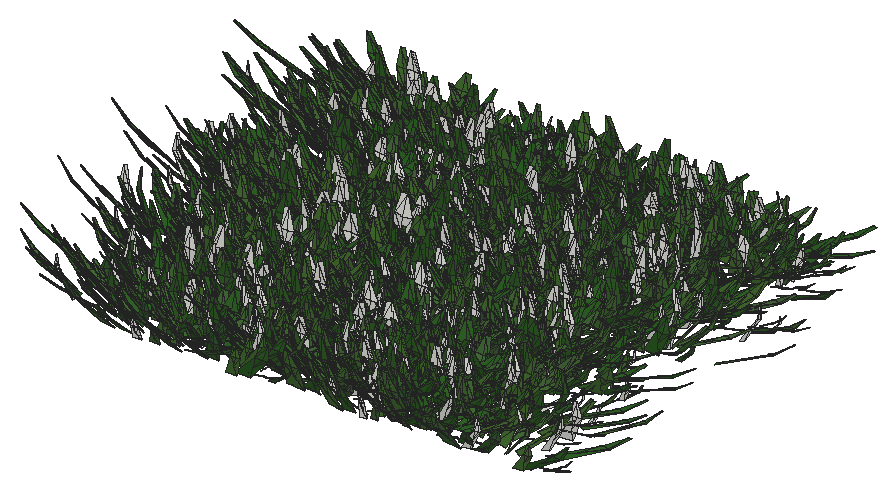
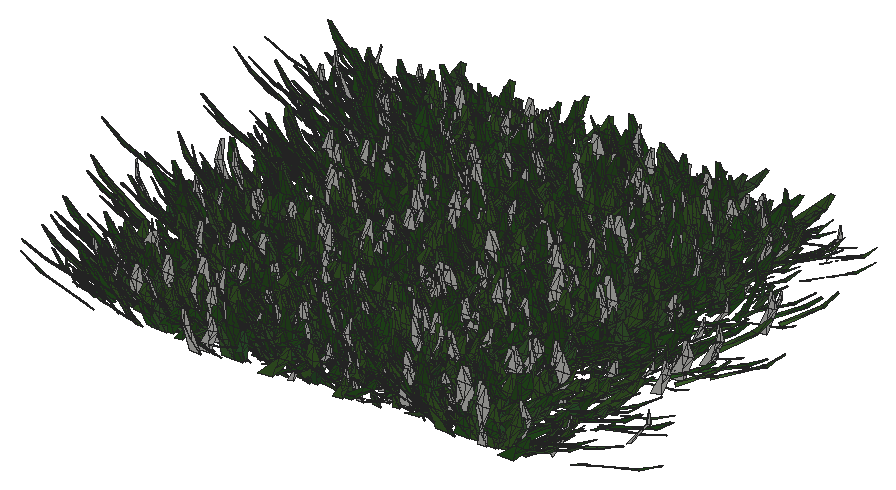
# SketchUp Ruby script. Lengths in inches.
U = 1.inch
M = Sketchup.active_model
def pt(a) = Geom::Point3d.new(a.map { |v| v * U })
def face(e, loops, mat)
  f = e.add_face(loops[0].map { |a| pt(a) })
  loops[1..].each { |l| e.add_face(l.map { |a| pt(a) }).erase! }
  f.material = f.back_material = mat if mat
  f
end
# faces: each face lists its corners as indices into pts; further lists are holes
def faces(e, pts, list, mat = nil) = list.each { |f| face(e, (f[0].is_a?(Array) ? f : [f]).map { |l| l.map { |i| pts[i] } }, mat) }
# xy, xz, yz: faces in a plane at the given z, y or x. An outline is a flat list of corners, or four numbers for a rectangle; further outlines are holes
def ring(l) = l.size == 4 ? [[l[0], l[1]], [l[2], l[1]], [l[2], l[3]], [l[0], l[3]]] : l.each_slice(2).to_a
def flat(e, list, mat, &to3) = list.each { |f| face(e, (f[0].is_a?(Array) ? f : [f]).map { |l| ring(l).map { |u, v| to3.(u, v) } }, mat) }
def xy(e, z, list, mat = nil) = flat(e, list, mat) { |x, y| [x, y, z] }
def xz(e, y, list, mat = nil) = flat(e, list, mat) { |x, z| [x, y, z] }
def yz(e, x, list, mat = nil) = flat(e, list, mat) { |y, z| [x, y, z] }
def lines(e, pts, list) = list.each { |a, b| e.add_line(pt(pts[a]), pt(pts[b])) }
# prism: a flat outline (further loops are holes) pulled along v
def prism(e, loops, v, mat = nil)
  f = face(e, loops, mat); d = Geom::Vector3d.new(v.map { |x| x * U })
  f.pushpull(f.normal.samedirection?(d) ? d.length : -d.length)
end
def box(e, o, s, mat = nil) = prism(e, [[o, [o[0] + s[0], o[1], o[2]], [o[0] + s[0], o[1] + s[1], o[2]], [o[0], o[1] + s[1], o[2]]]], [0, 0, s[2]], mat)
def at(x, y, z, deg = 0) = Geom::Transformation.translation(pt([x, y, z])) * Geom::Transformation.rotation(ORIGIN, Z_AXIS, deg.degrees)
def axes(o, x, y, z) = Geom::Transformation.new([*x, 0, *y, 0, *z, 0, *pt(o).to_a, 1])
def part(name) = M.definitions.add(name)
# library, detail: a bought-in or finely detailed component or shape, given as its bounding box
def library(name, o, s) = part(name).tap { |d| box(d.entities, o, s) }
def detail(e, o, s) = box(e.add_group.entities, o, s)
def put(e, d, t, mat = nil) = e.add_instance(d, t).tap { |i| i.material = mat if mat }
def group(e, t, mat = nil) = e.add_group.tap { |g| g.transformation = t; g.material = mat if mat }.entities
root = M.entities
M.materials.add("Material10").color = [48, 100, 38]
M.materials.add("Material3").color = [68, 110, 58]
M.materials.add("Material4").color = [48, 90, 38]
M.materials.add("Material5").color = [68, 110, 48]
M.materials.add("Material6").color = [48, 90, 48]
M.materials.add("Material7").color = [58, 110, 58]
M.materials.add("Material8").color = [58, 90, 38]
M.materials.add("Material9").color = [68, 100, 58]
c1 = part("grass00")
p = [[-0.6875,0.15,0],[-0.56,0.08,5.52],[-0.04,0.03,2.76],[0.48,-0.02,0],[0.35,-0.02,5.52],[-0.1,-0.14,5.52],
  [-0.12,0.65,8.37],[-0.42,0.65,8.37]]
faces(c1.entities,p,[[0,1,2,3],[3,2,4],[1,5,2],[5,4,2],[1,6,5],[4,5,6],[7,6,1]])
c2 = part("Group16\#1")
put(c2.entities,c1,axes([1.44,-0.61,-0.01],[0.05352,0.12609,0],[-0.10704,0.04543,0.07239],[0.06664,-0.02828,0.11628]),"Material6")
put(c2.entities,c1,axes([0.76,-0.15,-0.01],[0.04676,0.24062,0],[-0.23162,0.04501,0.06642],[0.0652,-0.01267,0.23595]),"Material3")
put(c2.entities,c1,axes([0.79,0.01,-0.01],[-0.00606,0.34651,0],[-0.34381,-0.00602,0.0432],[0.04319,0.00076,0.34386]))
put(c2.entities,c1,axes([1,0.23,-0.01],[-0.07192,0.31144,0],[-0.28722,-0.06632,0.1236],[0.12043,0.02781,0.29478]),"Material5")
put(c2.entities,c1,axes([1.66,0.77,-0.01],[-0.13828,0.29651,0],[-0.21551,-0.1005,0.22471],[0.20365,0.09498,0.23779]),"Material10")
put(c2.entities,c1,axes([0.6875,0.52,-0.01],[-0.18126,0.24051,0],[-0.22746,-0.17142,0.09788],[0.07817,0.05891,0.28481]),"Material5")
put(c2.entities,c1,axes([0.68,0.78,-0.01],[-0.215,0.18688,0],[-0.12385,-0.14248,0.21334],[0.13995,0.16101,0.18878]),"Material3")
put(c2.entities,c1,axes([0.56,1,-0.01],[-0.13756,0.07624,0],[-0.06159,-0.11112,0.0927],[0.04494,0.08108,0.12705]),"Material5")
put(c2.entities,c1,axes([0.2,0.64,-0.01],[-0.23729,0.07254,0],[-0.05711,-0.18681,0.153],[0.04473,0.14632,0.19535]),"Material10")
put(c2.entities,c1,axes([0.0625,0.72,-0.01],[-0.28874,0.02525,0],[-0.02179,-0.24916,0.14647],[0.01276,0.14591,0.25012]),"Material3")
put(c2.entities,c1,axes([-0.08,0.62,-0.01],[-0.34089,-0.04187,0],[0.03255,-0.26504,0.216],[-0.02633,0.21439,0.26703]),"Material10")
put(c2.entities,c1,axes([-0.34,0.98,-0.01],[-0.14314,-0.0493,0],[0.04397,-0.12769,0.06843],[-0.02228,0.0647,0.13505]),"Material10")
put(c2.entities,c1,axes([-0.87,1.45,-0.01],[-0.23488,-0.14114,0],[0.13761,-0.22901,0.06087],[-0.03135,0.05217,0.26717]))
put(c2.entities,c1,axes([-0.72,0.77,-0.01],[-0.14208,-0.13251,0],[0.07209,-0.0773,0.16301],[-0.11118,0.11922,0.1057]),"Material10")
put(c2.entities,c1,axes([-0.62,0.43,-0.01],[-0.14845,-0.21203,0],[0.18654,-0.13061,0.12304],[-0.10079,0.07057,0.22772]),"Material3")
put(c2.entities,c1,axes([-0.68,0.29,-0.01],[-0.13639,-0.32136,0],[0.31723,-0.13464,0.05579],[-0.05136,0.0218,0.34462]),"Material4")
put(c2.entities,c1,axes([-0.64,0.125,-0.01],[-0.0458,-0.23569,0],[0.22124,-0.043,0.08276],[-0.08124,0.01579,0.22538]),"Material7")
put(c2.entities,c1,axes([-1.6,-0.03,-0.01],[0.00576,-0.32897,0],[0.27526,0.00482,0.18018],[-0.18015,-0.00315,0.2753]),"Material5")
put(c2.entities,c1,axes([-1.36,-0.31,-0.01],[0.05718,-0.24765,0],[0.18172,0.04196,0.17267],[-0.16825,-0.03885,0.1865]),"Material10")
put(c2.entities,c1,axes([-1.54,-0.72,-0.01],[0.06537,-0.14017,0],[0.13555,0.06321,0.03939],[-0.0357,-0.01665,0.14956]))
put(c2.entities,c1,axes([-1.19,-0.9,-0.01],[0.09597,-0.12735,0],[0.11214,0.08451,0.07557],[-0.06035,-0.04548,0.14042]),"Material9")
put(c2.entities,c1,axes([-0.47,-0.54,-0.01],[0.11588,-0.10072,0],[0.0618,0.0711,0.12124],[-0.07953,-0.0915,0.0942]))
put(c2.entities,c1,axes([-0.47,-0.84,-0.01],[0.11927,-0.0661,0],[0.06603,0.11913,0.00646],[-0.00313,-0.00565,0.13621]),"Material5")
put(c2.entities,c1,axes([-0.38,-1.24,-0.01],[0.28037,-0.08571,0],[0.0618,0.20215,0.20315],[-0.05939,-0.19428,0.21139]),"Material9")
put(c2.entities,c1,axes([-0.06,-0.66,-0.01],[0.22719,-0.01987,0],[0.01247,0.14255,0.17758],[-0.01547,-0.17691,0.1431]),"Material8")
put(c2.entities,c1,axes([0.11,-0.89,-0.01],[0.14882,0.01828,0],[-0.01058,0.08611,0.12229],[0.01491,-0.12138,0.08676]),"Material6")
put(c2.entities,c1,axes([0.25,-0.72,-0.01],[0.20481,0.07053,0],[-0.06206,0.18022,0.10291],[0.03351,-0.0973,0.1906]),"Material6")
put(c2.entities,c1,axes([0.85,-1.42,-0.01],[0.16481,0.09904,0],[-0.09472,0.15762,0.05616],[0.02893,-0.04814,0.18389]),"Material5")
put(c2.entities,c1,axes([1.01,-1.09,-0.01],[0.21858,0.20385,0],[-0.17495,0.1876,0.15339],[0.10462,-0.11218,0.25652]),"Material10")
put(c2.entities,c1,axes([1.01,-0.71,-0.01],[0.08733,0.12473,0],[-0.06445,0.04512,0.13037],[0.1068,-0.07477,0.07867]),"Material6")
c3 = part("Group15\#1")
put(c3.entities,c2,at(0,0,0))
c4 = part("3darcstudiotree_grass00\#1")
put(c4.entities,c3,at(0,0,0))
put(root,c4,axes([1060.05,905.06,0],[3.81718,0.38538,0],[-1.70529,1.05566,-0.03343],[-0.08298,0.05137,1.88641]))
put(root,c4,axes([1060.56,931.82,0],[-0.16779,1.03236,0],[-3.91072,-0.03973,-0.03031],[-0.21719,-0.00221,1.75443]))
put(root,c4,axes([1060.23,917.13,0],[3.62954,0.33152,0],[-1.65878,1.13506,-0.04863],[-0.08609,0.05891,1.5585]))
put(root,c4,axes([1061.57,930.84,0],[-4.32193,0.57757,0],[-2.28366,-1.06804,-0.02635],[-0.05701,-0.02666,1.3895]))
put(root,c4,axes([1060.06,925.65,0],[2.41826,1.00361,0],[-4.45314,0.67064,-0.01693],[-0.07141,0.01075,1.59984]))
put(root,c4,axes([1060.86,914.74,0],[4.97151,0.37477,0],[-1.19031,0.98689,-0.04516],[-0.09125,0.07566,1.80387]))
put(root,c4,axes([1061.64,923.72,0],[-2.49241,1.02032,0],[-4.21954,-0.64421,-0.0342],[-0.15461,-0.0236,1.63693]))
put(root,c4,axes([1061.28,912.34,0],[3.70549,0.72715,0],[-2.49617,0.79502,-0.02005],[-0.09119,0.02904,1.86077]))
put(root,c4,axes([1063.53,931.57,0],[0.01218,-1.00906,0],[4.98185,0.00376,-0.03692],[0.18714,0.00014,1.57831]))
put(root,c4,axes([1063.89,916.37,0],[-1.42025,-0.83489,0],[4.16242,-0.44255,-0.01791],[0.11075,-0.01178,1.89984]))
put(root,c4,axes([1064.01,901.35,0],[0.28027,-0.96199,0],[3.64955,0.06646,-0.00937],[0.0792,0.00144,1.93766]))
put(root,c4,axes([1063.89,898.16,0],[-3.43805,0.34453,0],[-1.648,-1.02783,-0.04281],[-0.10438,-0.0651,1.81418]))
put(root,c4,axes([1063.77,927.84,0],[3.40925,-0.75567,0],[3.0298,0.85432,-0.03392],[0.10448,0.02946,1.32537]))
put(root,c4,axes([1064.98,905.9,0],[-4.27926,0.10077,0],[-0.4125,-1.0948,-0.0202],[-0.01348,-0.03577,1.95637]))
put(root,c4,axes([1063.73,894.94,0],[3.9837,-0.03206,0],[0.11597,0.90077,-0.04101],[0.00803,0.06239,1.37186]))
put(root,c4,axes([1064.41,930.31,0],[-2.74206,0.64257,0],[-3.29567,-0.87899,-0.02311],[-0.07278,-0.01941,1.38694]))
put(root,c4,axes([1065.68,925.63,0],[-4.52462,0.16915,0],[-0.75823,-1.26762,-0.06496],[-0.05656,-0.09455,1.88637]))
put(root,c4,axes([1064.79,913.76,0],[-1.87065,0.77621,0],[-4.34622,-0.65464,-0.04504],[-0.23728,-0.03574,1.9506]))
put(root,c4,axes([1065,920.09,0],[4.16044,-0.73269,0],[2.40364,0.85303,-0.03692],[0.14968,0.05312,1.83631]))
put(root,c4,axes([1064.86,896.66,0],[3.59915,0.14594,0],[-0.59052,0.91023,-0.01255],[-0.01426,0.02198,1.63564]))
put(root,c4,axes([1065.52,924.38,0],[-2.60039,0.90097,0],[-2.99223,-0.53976,-0.00844],[-0.04191,-0.00756,1.41311]))
put(root,c4,axes([1064.78,918.18,0],[2.59672,0.84047,0],[-3.92214,0.75737,-0.04605],[-0.16947,0.03272,1.44046]))
put(root,c4,axes([1066.125,907.85,0],[1.82286,-0.79645,0],[3.62821,0.519,-0.04415],[0.29175,0.04173,1.98924]))
put(root,c4,axes([1067.33,928.83,0],[-0.69021,-1.10068,0],[5.10027,-0.19989,-0.06318],[0.26987,-0.01058,1.39517]))
put(root,c4,axes([1065.64,908.85,0],[2.76483,1.10064,0],[-3.85856,0.6058,-0.052],[-0.27462,0.04312,1.7759]))
put(root,c4,axes([1066.5,923.28,0],[3.65122,-0.89135,0],[3.24538,0.83087,-0.04175],[0.1632,0.04178,1.62422]))
put(root,c4,axes([1065.84,920.87,0],[4.36658,0.08239,0],[-0.38033,1.25977,-0.00004],[-0.00002,0.00006,1.93334]))
put(root,c4,axes([1067.64,903.13,0],[-2.28283,-1.06843,0],[4.21309,-0.56261,-0.05822],[0.33198,-0.04433,1.92982]))
put(root,c4,axes([1066.68,914.86,0],[0.26997,1.23611,0],[-4.58463,0.06258,-0.05861],[-0.40129,0.00548,1.96776]))
put(root,c4,axes([1066.15,911.15,0],[4.48895,0.48675,0],[-1.69756,0.97846,-0.01845],[-0.03711,0.02139,1.34771]))
put(root,c4,axes([1066.18,894.22,0],[2.13817,1.11793,0],[-4.20741,0.50295,-0.01048],[-0.04572,0.00547,1.40926]))
put(root,c4,axes([1066.53,904.47,0],[4.31033,0.25907,0],[-1.20979,1.25799,-0.03506],[-0.03358,0.03491,1.32515]))
put(root,c4,axes([1067.25,900.07,0],[4.12313,-0.24157,0],[1.18082,1.25966,-0.02268],[0.02474,0.0264,1.5468]))
put(root,c4,axes([1067.24,911.875,0],[-0.03316,1.25701,0],[-4.94993,-0.00816,-0.01347],[-0.06338,-0.0001,1.45625]))
put(root,c4,axes([1069.67,899.01,0],[3.15531,-0.58243,0],[2.70786,0.91686,-0.02283],[0.06907,0.02339,1.4512]))
put(root,c4,axes([1070.67,902.47,0],[-1.85827,-1.20054,0],[4.6379,-0.44867,-0.05475],[0.3098,-0.02997,1.88574]))
put(root,c4,axes([1069.67,897,0],[3.52758,-0.61527,0],[2.26758,0.81256,-0.00731],[0.03042,0.0109,1.80073]))
put(root,c4,axes([1070.9,931.73,0],[-2.08937,-0.99009,0],[3.80908,-0.50239,-0.03938],[0.17969,-0.0237,1.38871]))
put(root,c4,axes([1069.88,922.42,0],[3.90144,-0.65649,0],[2.04826,0.76078,-0.0013],[0.00472,0.00175,1.49257]))
put(root,c4,axes([1069.77,904.9,0],[-1.15605,0.94536,0],[-4.28561,-0.32755,-0.0271],[-0.16007,-0.01223,1.72974]))
put(root,c4,axes([1071.1875,899.8125,0],[-4.45544,0.35262,0],[-1.28974,-1.0185,-0.03323],[-0.0666,-0.05259,1.77353]))
put(root,c4,axes([1070.16,895.2,0],[4.66445,0.12304,0],[-0.40469,0.95886,-0.03171],[-0.02368,0.05611,1.71518]))
put(root,c4,axes([1071.92,906.49,0],[0.22891,-1.1855,0],[4.26581,0.05148,-0.00402],[0.01994,0.00024,1.3243]))
put(root,c4,axes([1072.04,910.74,0],[-3.83276,-0.4307,0],[1.47756,-0.82179,-0.02079],[0.061,-0.03393,1.61237]))
put(root,c4,axes([1071.23,912.24,0],[-2.46367,0.88426,0],[-3.17691,-0.55321,-0.01437],[-0.09353,-0.01629,1.91898]))
put(root,c4,axes([1072.21,927.79,0],[-2.3426,-0.88357,0],[3.5724,-0.59197,-0.05028],[0.30493,-0.05053,1.94898]))
put(root,c4,axes([1070.97,930.54,0],[4.40447,-0.22368,0],[0.75254,0.92613,-0.00331],[0.00443,0.00545,1.58887]))
put(root,c4,axes([1070.42,921.03,0],[4.73855,0.38676,0],[-1.49783,1.14695,-0.00124],[-0.0021,0.00161,1.65228]))
put(root,c4,axes([1071.73,926.16,0],[-1.79093,0.80578,0],[-3.73339,-0.51862,-0.05151],[-0.32129,-0.04463,1.90487]))
put(root,c4,axes([1070.86,924.13,0],[1.1144,0.95521,0],[-4.67069,0.34057,-0.00405],[-0.01733,0.00126,1.35389]))
put(root,c4,axes([1073.37,918.5,0],[-3.69018,-0.70839,0],[2.67455,-0.87078,-0.00705],[0.02875,-0.00936,1.8369]))
put(root,c4,axes([1072.42,919.6,0],[2.21238,-0.82212,0],[4.12079,0.69308,-0.06298],[0.2244,0.03774,1.33293]))
put(root,c4,axes([1071.57,894.17,0],[4.71925,-0.11324,0],[0.46781,1.21853,-0.01064],[0.0059,0.01536,1.77558]))
put(root,c4,axes([1073.51,929.0625,0],[-3.23059,-0.98889,0],[3.90689,-0.79771,-0.03335],[0.15229,-0.03109,1.85855]))
put(root,c4,axes([1072.875,915.7,0],[0.38736,-1.28995,0],[5.0857,0.09545,-0.06273],[0.38626,0.00725,1.9684]))
put(root,c4,axes([1072.43,901.1,0],[-1.91482,0.78597,0],[-3.52393,-0.53658,-0.03041],[-0.133,-0.02025,1.3205]))
put(root,c4,axes([1073.875,914.15,0],[-1.97779,-0.85605,0],[3.47193,-0.50134,-0.00817],[0.04391,-0.00634,1.55447]))
put(root,c4,axes([1073.05,916.17,0],[4.07935,-0.43346,0],[1.89845,1.11667,-0.00549],[0.0102,0.006,1.44062]))
put(root,c4,axes([1073.04,907.98,0],[4.37754,-0.30034,0],[1.33809,1.21894,-0.05143],[0.06212,0.05659,1.44218]))
put(root,c4,axes([1073,909.25,0],[-0.77459,1.02893,0],[-4.84534,-0.22797,-0.01956],[-0.11313,-0.00532,1.8138]))
put(root,c4,axes([1075.72,906.38,0],[-4.74279,0.28772,0],[-1.21823,-1.25511,-0.06662],[-0.06794,-0.07,1.39642]))
put(root,c4,axes([1076.68,899.54,0],[-3.58073,-0.35661,0],[1.83074,-1.1489,-0.00121],[0.00279,-0.00175,1.92636]))
put(root,c4,axes([1075.85,930.3125,0],[1.54312,-0.81512,0],[3.29472,0.38983,-0.04441],[0.34585,0.04092,1.96303]))
put(root,c4,axes([1076.66,927.34,0],[-0.36487,-0.9693,0],[3.80087,-0.08942,-0.04952],[0.26852,-0.00632,1.29958]))
put(root,c4,axes([1076.78,924.32,0],[-3.87388,0.80913,0],[-2.80413,-0.83909,-0.03098],[-0.11588,-0.03468,1.59479]))
put(root,c4,axes([1077.45,932.95,0],[-4.21097,-0.15572,0],[0.54772,-0.92572,-0.00812],[0.00706,-0.01193,1.3892]))
put(root,c4,axes([1076.93,920.93,0],[-3.28993,0.53414,0],[-2.35898,-0.90811,-0.04277],[-0.16039,-0.06174,1.86401]))
put(root,c4,axes([1076.34,901.25,0],[-0.64164,1.09647,0],[-3.76994,-0.13788,-0.02144],[-0.17386,-0.00636,1.9513]))
put(root,c4,axes([1076.9,915.71,0],[-3.33719,0.61695,0],[-2.63683,-0.89144,-0.01371],[-0.03862,-0.01306,1.31321]))
put(root,c4,axes([1076.34,929.21,0],[3.65959,-0.0096,0],[0.04442,1.05836,-0.01029],[0.00057,0.0135,1.389]))
put(root,c4,axes([1077.57,904.44,0],[1.63627,-0.81784,0],[3.89049,0.48648,-0.01805],[0.09406,0.01176,1.58457]))
put(root,c4,axes([1076.61,919.86,0],[4.2926,-0.51485,0],[1.76165,0.91799,-0.04597],[0.12323,0.06421,1.57738]))
put(root,c4,axes([1076.81,917.96,0],[-2.40518,0.923,0],[-4.34744,-0.70804,-0.00953],[-0.03635,-0.00592,1.47621]))
put(root,c4,axes([1078.18,931.99,0],[1.06062,-0.94983,0],[4.26034,0.29733,-0.00232],[0.01421,0.00099,1.76107]))
put(root,c4,axes([1077.08,922.95,0],[3.58152,-0.18688,0],[0.799,0.95704,-0.04941],[0.06002,0.07189,1.4533]))
put(root,c4,axes([1078.43,911.17,0],[2.30537,-0.84658,0],[3.6231,0.61664,-0.01892],[0.09951,0.01694,1.74337]))
put(root,c4,axes([1078.3,896.47,0],[-2.37312,0.89049,0],[-3.32471,-0.55376,-0.03773],[-0.17795,-0.02964,1.41517]))
put(root,c4,axes([1077.45,925.65,0],[4.42223,0.30333,0],[-1.18434,1.07915,-0.02738],[-0.04878,0.04444,1.88342]))
put(root,c4,axes([1078.06,916.16,0],[4.7526,-0.49648,0],[1.99217,1.19189,-0.05614],[0.10535,0.06303,1.57175]))
put(root,c4,axes([1079.17,908.06,0],[2.12632,-1.16665,0],[4.03974,0.46017,-0.02827],[0.17992,0.0205,1.94019]))
put(root,c4,axes([1078.41,912.15,0],[0.82616,1.18847,0],[-3.57688,0.1554,-0.03272],[-0.26216,0.01139,1.8454]))
put(root,c4,axes([1078.12,913.71,0],[3.22998,0.67416,0],[-3.0562,0.91516,-0.05497],[-0.20916,0.06263,1.76958]))
put(root,c4,axes([1078.09,908.5625,0],[2.39946,0.73907,0],[-3.00526,0.6098,-0.00448],[-0.02213,0.00449,1.5389]))
put(root,c4,axes([1079.36,903.23,0],[2.55238,-0.83938,0],[4.10588,0.78031,-0.05929],[0.21983,0.04178,1.50135]))
put(root,c4,axes([1079.08,895.41,0],[-0.55541,1.00886,0],[-4.55532,-0.15674,-0.0385],[-0.20653,-0.00711,1.55608]))
put(root,c4,axes([1079.5,898.66,0],[4.68045,-0.41888,0],[1.5867,1.1081,-0.05713],[0.0969,0.06767,1.48067]))
put(root,c4,axes([1081.74,925.4,0],[-3.20384,-1.02326,0],[3.97726,-0.7783,-0.01534],[0.06587,-0.01289,1.72134]))
put(root,c4,axes([1081.51,915.32,0],[-4.59803,0.08563,0],[-0.2847,-0.9555,-0.0204],[-0.00865,-0.02903,1.3669]))
put(root,c4,axes([1081.91,928.65,0],[-4.38136,-0.40254,0],[1.40005,-0.95241,-0.00277],[0.00519,-0.00353,1.38049]))
put(root,c4,axes([1082.49,917.03,0],[-3.71243,-0.56774,0],[2.64786,-1.08214,-0.03935],[0.09328,-0.03812,1.44076]))
put(root,c4,axes([1081.74,898.1875,0],[4.21231,-0.52689,0],[1.66569,0.83229,-0.01525],[0.04687,0.02342,1.59832]))
put(root,c4,axes([1082.43,921.26,0],[2.41687,-0.67519,0],[3.02095,0.67585,-0.01984],[0.10631,0.02378,1.82222]))
put(root,c4,axes([1082.23,917.8,0],[0.7487,1.19338,0],[-3.70978,0.14547,-0.03929],[-0.32325,0.01268,1.95437]))
put(root,c4,axes([1083.85,922.72,0],[-2.24094,-0.73195,0],[3.39914,-0.65043,-0.02737],[0.10576,-0.02024,1.30175]))
put(root,c4,axes([1082.67,913.375,0],[-0.31652,1.20504,0],[-3.66531,-0.06017,-0.03425],[-0.24045,-0.00395,1.61497]))
put(root,c4,axes([1083.59,927.59,0],[1.87547,-0.90536,0],[3.87003,0.50105,-0.01075],[0.05218,0.00676,1.48923]))
put(root,c4,axes([1083.89,904.1,0],[-4.13074,0.02619,0],[-0.11371,-1.1209,-0.00196],[-0.00027,-0.00262,1.49745]))
put(root,c4,axes([1083.17,900.21,0],[-2.5882,0.79848,0],[-3.68123,-0.74577,-0.04128],[-0.16563,-0.03355,1.52936]))
put(root,c4,axes([1082.7,903.26,0],[4.43719,0.0399,0],[-0.16058,1.11619,-0.02702],[-0.00694,0.04824,1.99535]))
put(root,c4,axes([1083.69,933.76,0],[2.51749,-0.66921,0],[3.09976,0.7288,-0.02136],[0.09486,0.0223,1.62144]))
put(root,c4,axes([1084.49,901.72,0],[-4.57103,-0.1339,0],[0.44169,-0.94237,-0.00847],[0.00759,-0.0162,1.82708]))
put(root,c4,axes([1083.34,920.07,0],[1.81154,0.83974,0],[-3.36309,0.45344,-0.03445],[-0.23344,0.03147,1.83855]))
put(root,c4,axes([1085.2,897.53,0],[-3.18482,-0.5306,0],[2.64212,-0.99117,-0.04785],[0.16263,-0.06101,1.82518]))
put(root,c4,axes([1084.13,911.13,0],[-1.1436,1.00471,0],[-3.56675,-0.25374,-0.00052],[-0.00362,-0.00026,1.67384]))
put(root,c4,axes([1084.28,911.89,0],[4.19446,0.12436,0],[-0.54634,1.15167,-0.05841],[-0.03094,0.06521,1.30397]))
put(root,c4,axes([1085.94,907.14,0],[-3.94605,-0.19743,0],[0.76142,-0.95114,-0.00178],[0.00253,-0.00316,1.75352]))
put(root,c4,axes([1085.34,924.06,0],[-3.21823,0.62251,0],[-2.5621,-0.82785,-0.04163],[-0.13582,-0.04388,1.39503]))
put(root,c4,axes([1084.4,930.07,0],[2.86514,0.59771,0],[-2.37877,0.71266,-0.00812],[-0.03621,0.01085,1.6158]))
put(root,c4,axes([1084.36,906.28,0],[2.40396,0.87072,0],[-3.51835,0.60711,-0.02215],[-0.11639,0.02008,1.70619]))
put(root,c4,axes([1085.09,894.92,0],[0.47461,1.07377,0],[-3.68217,0.10172,-0.03685],[-0.27492,0.00759,1.73767]))
put(root,c4,axes([1084.68,931.33,0],[4.18661,0.73977,0],[-2.83874,1.00409,-0.0169],[-0.04607,0.01629,1.45184]))
put(root,c4,axes([1085.72,909.07,0],[4.09522,-0.17448,0],[0.64394,0.9446,-0.03176],[0.04135,0.06066,1.85682]))
put(root,c4,axes([1087.77,904.2,0],[-2.585,-1.04322,0],[3.07878,-0.47681,-0.00146],[0.00727,-0.00113,1.32424]))
put(root,c4,axes([1087.72,900.38,0],[4.12343,-0.57612,0],[2.31328,1.0348,-0.04605],[0.10519,0.04706,1.38783]))
put(root,c4,axes([1089.11,898.28,0],[-3.01934,-0.67461,0],[2.59527,-0.72597,-0.04195],[0.17887,-0.05004,1.55746]))
put(root,c4,axes([1087.54,930.23,0],[1.24737,1.15044,0],[-4.46094,0.3023,-0.03421],[-0.2215,0.01501,1.93796]))
put(root,c4,axes([1089.73,909.57,0],[-1.14351,-1.16914,0],[4.8405,-0.2959,-0.03172],[0.13527,-0.00827,1.36741]))
put(root,c4,axes([1089.9,895.48,0],[-3.21504,-0.48766,0],[2.28718,-0.94243,-0.00574],[0.01454,-0.00599,1.3472]))
put(root,c4,axes([1089.92,915.66,0],[-3.15035,-0.75707,0],[2.9131,-0.75763,-0.02949],[0.15297,-0.03979,1.96656]))
put(root,c4,axes([1090.08,919.45,0],[-3.24274,-0.9643,0],[3.00099,-0.63073,-0.02964],[0.15134,-0.03181,1.63454]))
put(root,c4,axes([1088.33,907.93,0],[3.01617,0.89347,0],[-2.94209,0.62075,-0.05003],[-0.28997,0.06118,1.82479]))
put(root,c4,axes([1088.52,912.24,0],[2.5933,0.94523,0],[-3.23927,0.55545,-0.03781],[-0.2219,0.03805,1.74723]))
put(root,c4,axes([1088.58,931.83,0],[4.89603,0.07684,0],[-0.28824,1.14785,-0.04601],[-0.01316,0.0524,1.31249]))
put(root,c4,axes([1089.28,918.3,0],[-2.72717,0.91933,0],[-3.49968,-0.64886,-0.0152],[-0.05921,-0.01098,1.3203]))
put(root,c4,axes([1088.68,913.11,0],[1.14482,1.02843,0],[-4.70727,0.3275,-0.02844],[-0.16339,0.01137,1.82107]))
put(root,c4,axes([1089.53,927.34,0],[-2.54341,1.08635,0],[-4.03419,-0.59031,-0.03733],[-0.16382,-0.02397,1.48568]))
put(root,c4,axes([1088.86,923.77,0],[2.27146,0.75873,0],[-3.43794,0.64327,-0.0157],[-0.07531,0.01409,1.60759]))
put(root,c4,axes([1089.625,910.19,0],[3.97684,-0.65785,0],[2.37523,0.89742,-0.03005],[0.11618,0.04389,1.88475]))
put(root,c4,axes([1089.18,917.22,0],[0.9962,1.21765,0],[-4.18163,0.21382,-0.01369],[-0.07051,0.00361,1.40267]))
put(root,c4,axes([1089.83,897.03,0],[0.30444,1.1436,0],[-4.22382,0.07028,-0.01024],[-0.07034,0.00117,1.82096]))
put(root,c4,axes([1090.38,922.1875,0],[-1.34742,1.17452,0],[-4.20278,-0.30134,-0.02925],[-0.13999,-0.01004,1.36051]))
put(root,c4,axes([1090.01,926.09,0],[2.73951,0.74881,0],[-3.24608,0.74223,-0.03451],[-0.17558,0.04015,1.89576]))
put(root,c4,axes([1090.17,929.125,0],[4.21944,0.50022,0],[-1.55878,0.82178,-0.0026],[-0.00889,0.00468,1.81639]))
put(root,c4,axes([1091.875,903.1,0],[-4.32099,0.14556,0],[-0.59248,-1.09927,-0.01091],[-0.0098,-0.01818,1.8656]))
put(root,c4,axes([1090.39,901,0],[5.12297,0.07434,0],[-0.27761,1.19572,-0.0212],[-0.00806,0.03474,1.96575]))
put(root,c4,axes([1090.71,920.96,0],[4.26894,0.36032,0],[-1.62732,1.205,-0.0473],[-0.09046,0.06698,1.90097]))
put(root,c4,axes([1090.77,933.67,0],[4.07758,0.30015,0],[-1.15535,0.98096,-0.01058],[-0.01796,0.01525,1.53588]))
put(root,c4,axes([1090.96,906.03,0],[3.97096,0.2686,0],[-1.03044,0.95214,-0.04799],[-0.08149,0.0753,1.60328]))
put(root,c4,axes([1094.34,898.68,0],[-3.00965,-0.629,0],[2.74401,-0.82061,-0.04185],[0.17493,-0.05231,1.7425]))
put(root,c4,axes([1094.65,920.91,0],[-2.42345,-0.78583,0],[3.59047,-0.69205,-0.03514],[0.17335,-0.03341,1.76492]))
put(root,c4,axes([1094.58,928.78,0],[1.70921,-0.84435,0],[3.84914,0.48698,-0.00728],[0.03207,0.00406,1.33141]))
put(root,c4,axes([1094.02,930.25,0],[-1.51485,1.06951,0],[-3.50861,-0.3106,-0.04758],[-0.30375,-0.02689,1.57537]))
put(root,c4,axes([1095.17,901.56,0],[-4.50974,-0.37005,0],[1.35893,-1.03507,-0.0393],[0.07695,-0.05861,1.71017]))
put(root,c4,axes([1094.7,923.08,0],[-4.37049,0.5936,0],[-1.84843,-0.85059,-0.00649],[-0.01819,-0.00837,1.42064]))
put(root,c4,axes([1093.99,932,0],[-0.14514,1.16082,0],[-3.94632,-0.03084,-0.04056],[-0.22687,-0.00177,1.38085]))
put(root,c4,axes([1094.92,908.55,0],[-2.03317,0.85161,0],[-3.54583,-0.52909,-0.0186],[-0.09087,-0.01356,1.46845]))
put(root,c4,axes([1095.11,916.13,0],[3.9809,-0.25729,0],[1.14083,1.10321,-0.04398],[0.07296,0.07055,1.88821]))
put(root,c4,axes([1095.06,895.69,0],[4.79923,0.3708,0],[-1.47799,1.19558,-0.04987],[-0.07603,0.0615,1.61513]))
